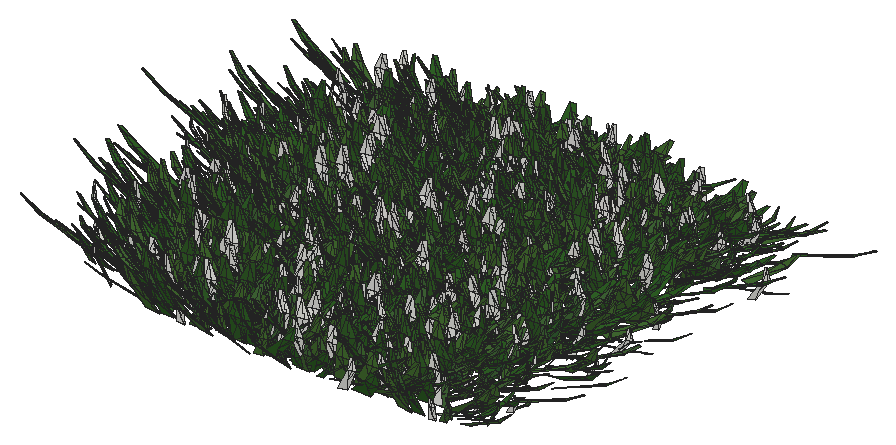
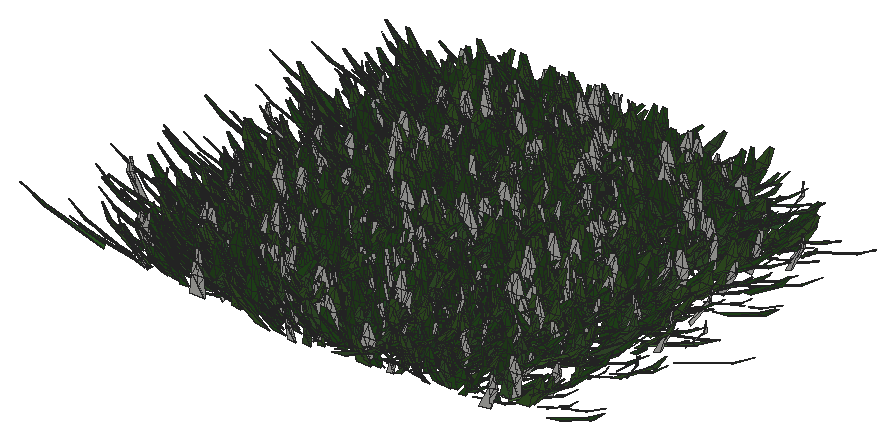
# SketchUp Ruby script. Lengths in inches.
U = 1.inch
M = Sketchup.active_model
def pt(a) = Geom::Point3d.new(a.map { |v| v * U })
def face(e, loops, mat)
  f = e.add_face(loops[0].map { |a| pt(a) })
  loops[1..].each { |l| e.add_face(l.map { |a| pt(a) }).erase! }
  f.material = f.back_material = mat if mat
  f
end
# faces: each face lists its corners as indices into pts; further lists are holes
def faces(e, pts, list, mat = nil) = list.each { |f| face(e, (f[0].is_a?(Array) ? f : [f]).map { |l| l.map { |i| pts[i] } }, mat) }
# xy, xz, yz: faces in a plane at the given z, y or x. An outline is a flat list of corners, or four numbers for a rectangle; further outlines are holes
def ring(l) = l.size == 4 ? [[l[0], l[1]], [l[2], l[1]], [l[2], l[3]], [l[0], l[3]]] : l.each_slice(2).to_a
def flat(e, list, mat, &to3) = list.each { |f| face(e, (f[0].is_a?(Array) ? f : [f]).map { |l| ring(l).map { |u, v| to3.(u, v) } }, mat) }
def xy(e, z, list, mat = nil) = flat(e, list, mat) { |x, y| [x, y, z] }
def xz(e, y, list, mat = nil) = flat(e, list, mat) { |x, z| [x, y, z] }
def yz(e, x, list, mat = nil) = flat(e, list, mat) { |y, z| [x, y, z] }
def lines(e, pts, list) = list.each { |a, b| e.add_line(pt(pts[a]), pt(pts[b])) }
# prism: a flat outline (further loops are holes) pulled along v
def prism(e, loops, v, mat = nil)
  f = face(e, loops, mat); d = Geom::Vector3d.new(v.map { |x| x * U })
  f.pushpull(f.normal.samedirection?(d) ? d.length : -d.length)
end
def box(e, o, s, mat = nil) = prism(e, [[o, [o[0] + s[0], o[1], o[2]], [o[0] + s[0], o[1] + s[1], o[2]], [o[0], o[1] + s[1], o[2]]]], [0, 0, s[2]], mat)
def at(x, y, z, deg = 0) = Geom::Transformation.translation(pt([x, y, z])) * Geom::Transformation.rotation(ORIGIN, Z_AXIS, deg.degrees)
def axes(o, x, y, z) = Geom::Transformation.new([*x, 0, *y, 0, *z, 0, *pt(o).to_a, 1])
def part(name) = M.definitions.add(name)
# library, detail: a bought-in or finely detailed component or shape, given as its bounding box
def library(name, o, s) = part(name).tap { |d| box(d.entities, o, s) }
def detail(e, o, s) = box(e.add_group.entities, o, s)
def put(e, d, t, mat = nil) = e.add_instance(d, t).tap { |i| i.material = mat if mat }
def group(e, t, mat = nil) = e.add_group.tap { |g| g.transformation = t; g.material = mat if mat }.entities
root = M.entities
M.materials.add("Material10").color = [48, 100, 38]
M.materials.add("Material3").color = [68, 110, 58]
M.materials.add("Material4").color = [48, 90, 38]
M.materials.add("Material5").color = [68, 110, 48]
M.materials.add("Material6").color = [48, 90, 48]
M.materials.add("Material7").color = [58, 110, 58]
M.materials.add("Material8").color = [58, 90, 38]
M.materials.add("Material9").color = [68, 100, 58]
c1 = part("grass00")
p = [[-0.6875,0.15,0],[-0.56,0.08,5.52],[-0.04,0.03,2.76],[0.48,-0.02,0],[0.35,-0.02,5.52],[-0.1,-0.14,5.52],
  [-0.12,0.65,8.37],[-0.42,0.65,8.37]]
faces(c1.entities,p,[[0,1,2,3],[3,2,4],[1,5,2],[5,4,2],[1,6,5],[4,5,6],[7,6,1]])
c2 = part("Group16\#1")
put(c2.entities,c1,axes([1.44,-0.61,-0.01],[0.05352,0.12609,0],[-0.10704,0.04543,0.07239],[0.06664,-0.02828,0.11628]),"Material6")
put(c2.entities,c1,axes([0.76,-0.15,-0.01],[0.04676,0.24062,0],[-0.23162,0.04501,0.06642],[0.0652,-0.01267,0.23595]),"Material3")
put(c2.entities,c1,axes([0.79,0.01,-0.01],[-0.00606,0.34651,0],[-0.34381,-0.00602,0.0432],[0.04319,0.00076,0.34386]))
put(c2.entities,c1,axes([1,0.23,-0.01],[-0.07192,0.31144,0],[-0.28722,-0.06632,0.1236],[0.12043,0.02781,0.29478]),"Material5")
put(c2.entities,c1,axes([1.66,0.77,-0.01],[-0.13828,0.29651,0],[-0.21551,-0.1005,0.22471],[0.20365,0.09498,0.23779]),"Material10")
put(c2.entities,c1,axes([0.6875,0.52,-0.01],[-0.18126,0.24051,0],[-0.22746,-0.17142,0.09788],[0.07817,0.05891,0.28481]),"Material5")
put(c2.entities,c1,axes([0.68,0.78,-0.01],[-0.215,0.18688,0],[-0.12385,-0.14248,0.21334],[0.13995,0.16101,0.18878]),"Material3")
put(c2.entities,c1,axes([0.56,1,-0.01],[-0.13756,0.07624,0],[-0.06159,-0.11112,0.0927],[0.04494,0.08108,0.12705]),"Material5")
put(c2.entities,c1,axes([0.2,0.64,-0.01],[-0.23729,0.07254,0],[-0.05711,-0.18681,0.153],[0.04473,0.14632,0.19535]),"Material10")
put(c2.entities,c1,axes([0.0625,0.72,-0.01],[-0.28874,0.02525,0],[-0.02179,-0.24916,0.14647],[0.01276,0.14591,0.25012]),"Material3")
put(c2.entities,c1,axes([-0.08,0.62,-0.01],[-0.34089,-0.04187,0],[0.03255,-0.26504,0.216],[-0.02633,0.21439,0.26703]),"Material10")
put(c2.entities,c1,axes([-0.34,0.98,-0.01],[-0.14314,-0.0493,0],[0.04397,-0.12769,0.06843],[-0.02228,0.0647,0.13505]),"Material10")
put(c2.entities,c1,axes([-0.87,1.45,-0.01],[-0.23488,-0.14114,0],[0.13761,-0.22901,0.06087],[-0.03135,0.05217,0.26717]))
put(c2.entities,c1,axes([-0.72,0.77,-0.01],[-0.14208,-0.13251,0],[0.07209,-0.0773,0.16301],[-0.11118,0.11922,0.1057]),"Material10")
put(c2.entities,c1,axes([-0.62,0.43,-0.01],[-0.14845,-0.21203,0],[0.18654,-0.13061,0.12304],[-0.10079,0.07057,0.22772]),"Material3")
put(c2.entities,c1,axes([-0.68,0.29,-0.01],[-0.13639,-0.32136,0],[0.31723,-0.13464,0.05579],[-0.05136,0.0218,0.34462]),"Material4")
put(c2.entities,c1,axes([-0.64,0.125,-0.01],[-0.0458,-0.23569,0],[0.22124,-0.043,0.08276],[-0.08124,0.01579,0.22538]),"Material7")
put(c2.entities,c1,axes([-1.6,-0.03,-0.01],[0.00576,-0.32897,0],[0.27526,0.00482,0.18018],[-0.18015,-0.00315,0.2753]),"Material5")
put(c2.entities,c1,axes([-1.36,-0.31,-0.01],[0.05718,-0.24765,0],[0.18172,0.04196,0.17267],[-0.16825,-0.03885,0.1865]),"Material10")
put(c2.entities,c1,axes([-1.54,-0.72,-0.01],[0.06537,-0.14017,0],[0.13555,0.06321,0.03939],[-0.0357,-0.01665,0.14956]))
put(c2.entities,c1,axes([-1.19,-0.9,-0.01],[0.09597,-0.12735,0],[0.11214,0.08451,0.07557],[-0.06035,-0.04548,0.14042]),"Material9")
put(c2.entities,c1,axes([-0.47,-0.54,-0.01],[0.11588,-0.10072,0],[0.0618,0.0711,0.12124],[-0.07953,-0.0915,0.0942]))
put(c2.entities,c1,axes([-0.47,-0.84,-0.01],[0.11927,-0.0661,0],[0.06603,0.11913,0.00646],[-0.00313,-0.00565,0.13621]),"Material5")
put(c2.entities,c1,axes([-0.38,-1.24,-0.01],[0.28037,-0.08571,0],[0.0618,0.20215,0.20315],[-0.05939,-0.19428,0.21139]),"Material9")
put(c2.entities,c1,axes([-0.06,-0.66,-0.01],[0.22719,-0.01987,0],[0.01247,0.14255,0.17758],[-0.01547,-0.17691,0.1431]),"Material8")
put(c2.entities,c1,axes([0.11,-0.89,-0.01],[0.14882,0.01828,0],[-0.01058,0.08611,0.12229],[0.01491,-0.12138,0.08676]),"Material6")
put(c2.entities,c1,axes([0.25,-0.72,-0.01],[0.20481,0.07053,0],[-0.06206,0.18022,0.10291],[0.03351,-0.0973,0.1906]),"Material6")
put(c2.entities,c1,axes([0.85,-1.42,-0.01],[0.16481,0.09904,0],[-0.09472,0.15762,0.05616],[0.02893,-0.04814,0.18389]),"Material5")
put(c2.entities,c1,axes([1.01,-1.09,-0.01],[0.21858,0.20385,0],[-0.17495,0.1876,0.15339],[0.10462,-0.11218,0.25652]),"Material10")
put(c2.entities,c1,axes([1.01,-0.71,-0.01],[0.08733,0.12473,0],[-0.06445,0.04512,0.13037],[0.1068,-0.07477,0.07867]),"Material6")
c3 = part("Group15\#1")
put(c3.entities,c2,at(0,0,0))
c4 = part("3darcstudiotree_grass00\#1")
put(c4.entities,c3,at(0,0,0))
put(root,c4,axes([159.55,67.09,7.6],[-4.17134,0.59694,0],[-1.91655,-0.83704,-0.03218],[-0.1099,-0.048,1.65786]))
put(root,c4,axes([160.14,46.88,7.6],[1.82974,-1.11236,0],[4.14269,0.4259,-0.00107],[0.00497,0.00051,1.41133]))
put(root,c4,axes([159.38,79.67,7.6],[-2.1717,0.94775,0],[-3.61053,-0.51708,-0.00674],[-0.03293,-0.00472,1.46389]))
put(root,c4,axes([159.7,53.77,7.6],[-1.78952,0.96069,0],[-3.60864,-0.42012,-0.01596],[-0.10849,-0.01263,1.86544]))
put(root,c4,axes([159.95,57.98,7.6],[-2.06309,0.87153,0],[-4.13288,-0.61146,-0.04665],[-0.19777,-0.02926,1.47851]))
put(root,c4,axes([161.13,74.04,7.6],[-3.51429,-0.45659,0],[1.66461,-0.80077,-0.02241],[0.07721,-0.03714,1.68548]))
put(root,c4,axes([160.16,66.55,7.6],[2.73197,0.7121,0],[-2.97454,0.71324,-0.02632],[-0.14399,0.03453,1.95302]))
put(root,c4,axes([160.55,71.85,7.6],[4.48019,-0.41485,0],[1.31658,0.88866,-0.03178],[0.08406,0.05674,1.80429]))
put(root,c4,axes([160.35,49.35,7.6],[2.54094,0.64898,0],[-3.14239,0.76896,-0.01876],[-0.08636,0.02113,1.77063]))
put(root,c4,axes([161.15,62.51,7.6],[0.1997,1.06432,0],[-4.51312,0.05293,-0.04808],[-0.29009,0.0034,1.70557]))
put(root,c4,axes([160.55,64.97,7.6],[1.85724,1.07697,0],[-4.66485,0.50278,-0.01792],[-0.06948,0.00749,1.34035]))
put(root,c4,axes([163.5,73.8125,7.6],[-1.0135,-1.00462,0],[4.08606,-0.25764,-0.02503],[0.13624,-0.00859,1.47852]))
put(root,c4,axes([162.99,53.55,7.6],[-4.005,0.7272,0],[-2.3018,-0.79231,-0.02785],[-0.12344,-0.04249,1.84622]))
put(root,c4,axes([162.97,61.53,7.6],[2.95335,-0.82152,0],[2.70823,0.6085,-0.01288],[0.06524,0.01466,1.54961]))
put(root,c4,axes([163.93,56.8125,7.6],[-4.20956,-0.26717,0],[1.18231,-1.16431,-0.00944],[0.01496,-0.01473,1.93444]))
put(root,c4,axes([163.76,52.31,7.6],[-1.13661,-1.06386,0],[4.15271,-0.27729,-0.04991],[0.23787,-0.01588,1.32514]))
put(root,c4,axes([163.9,51.05,7.6],[2.16693,-1.10955,0],[3.94511,0.48154,-0.03421],[0.21213,0.02589,1.89316]))
put(root,c4,axes([163.04,63.26,7.6],[1.18,1.03822,0],[-4.57121,0.32472,-0.01918],[-0.11705,0.00831,1.88463]))
put(root,c4,axes([164.6875,72.41,7.6],[-3.50507,0.61445,0],[-2.29769,-0.81919,-0.04222],[-0.17037,-0.06074,1.75818]))
put(root,c4,axes([165.76,69.23,7.6],[-3.58509,-0.60969,0],[2.592,-0.9526,-0.01911],[0.04957,-0.01822,1.32815]))
put(root,c4,axes([165.39,49.4,7.6],[-0.06451,-0.92143,0],[4.54272,-0.01988,-0.04239],[0.21245,-0.00093,1.42343]))
put(root,c4,axes([165.45,74.96,7.6],[-4.03446,-0.01635,0],[0.06659,-1.02672,-0.00434],[0.00038,-0.00582,1.37632]))
put(root,c4,axes([164.02,81.125,7.6],[3.92463,0.27646,0],[-1.34669,1.19487,-0.04858],[-0.06681,0.05928,1.57379]))
put(root,c4,axes([166.28,60.26,7.6],[-0.14207,-1.06089,0],[4.63971,-0.03883,-0.02714],[0.13515,-0.00113,1.44559]))
put(root,c4,axes([165.8,66.5,7.6],[-4.11295,0.48392,0],[-1.88318,-1.00036,-0.0027],[-0.00657,-0.00349,1.57765]))
put(root,c4,axes([165.86,79.88,7.6],[-3.01374,0.50325,0],[-2.28022,-0.85345,-0.04884],[-0.14675,-0.05493,1.38796]))
put(root,c4,axes([165.86,45.25,7.6],[2.85144,-0.93309,0],[3.29337,0.62902,-0.00592],[0.03247,0.0062,1.78738]))
put(root,c4,axes([166.8,45.98,7.6],[-2.85912,-0.7944,0],[3.18267,-0.71592,-0.02928],[0.11058,-0.02487,1.35967]))
put(root,c4,axes([167.0625,77.8,7.6],[-4.01975,-0.67401,0],[2.06418,-0.76941,-0.03319],[0.1306,-0.04868,1.63594]))
put(root,c4,axes([165.64,70.24,7.6],[-0.9226,1.08456,0],[-4.51637,-0.24012,-0.02719],[-0.16539,-0.00879,1.79436]))
put(root,c4,axes([165.94,64.02,7.6],[-0.15668,0.99341,0],[-4.74141,-0.04674,-0.01193],[-0.07952,-0.00078,1.97773]))
put(root,c4,axes([166.9,67.77,7.6],[-0.75974,1.09038,0],[-3.60462,-0.15698,-0.03897],[-0.29833,-0.01299,1.77692]))
put(root,c4,axes([166.78,55.85,7.6],[-0.10594,0.90385,0],[-3.73304,-0.02735,-0.04664],[-0.28296,-0.00207,1.41669]))
put(root,c4,axes([166.32,43.64,7.6],[1.08855,0.96574,0],[-4.18203,0.29461,-0.02067],[-0.12416,0.00875,1.69495]))
put(root,c4,axes([166.72,59,7.6],[3.05692,0.87665,0],[-2.75486,0.6004,-0.0286],[-0.17096,0.03726,1.81122]))
put(root,c4,axes([166.99,48.17,7.6],[-0.61059,1.1553,0],[-4.99702,-0.16506,-0.03274],[-0.14868,-0.00491,1.44297]))
put(root,c4,axes([166.8125,76.65,7.6],[4.02977,0.69816,0],[-2.76519,0.99754,-0.01195],[-0.03084,0.01113,1.37528]))
put(root,c4,axes([169.07,69.11,7.6],[-4.6224,0.20326,0],[-0.67084,-0.9535,-0.03096],[-0.03075,-0.04371,1.38775]))
put(root,c4,axes([169.28,58.54,7.6],[-3.52473,0.27582,0],[-1.46531,-1.17033,-0.0251],[-0.03902,-0.03117,1.59541]))
put(root,c4,axes([169.85,79.63,7.6],[-3.34559,-0.54215,0],[2.26075,-0.87194,-0.04254],[0.15941,-0.06148,1.78955]))
put(root,c4,axes([169.31,67.16,7.6],[-3.01586,0.58588,0],[-3.13511,-1.00864,-0.03993],[-0.14863,-0.04782,1.9372]))
put(root,c4,axes([170.27,71.76,7.6],[-4.50764,0.05804,0],[-0.237,-1.15033,-0.00589],[-0.00143,-0.00694,1.35922]))
put(root,c4,axes([169.34,49,7.6],[0.84914,1.0367,0],[-4.55233,0.23304,-0.02758],[-0.15102,0.00773,1.62317]))
put(root,c4,axes([171.27,81.41,7.6],[0.34339,-1.17076,0],[3.77324,0.06917,-0.00239],[0.01439,0.00026,1.42634]))
put(root,c4,axes([169.63,59.57,7.6],[0.91899,1.10711,0],[-4.12174,0.21384,-0.00381],[-0.02297,0.00119,1.62105]))
put(root,c4,axes([171.51,75.35,7.6],[-4.49867,-0.03279,0],[0.10809,-0.92683,-0.0193],[0.00484,-0.04152,1.99558]))
put(root,c4,axes([171.56,55.1,7.6],[-5.14292,0.15234,0],[-0.50377,-1.06293,-0.03012],[-0.01728,-0.03646,1.30483]))
put(root,c4,axes([170.37,46.2,7.6],[-1.72517,0.88368,0],[-4.30295,-0.52503,-0.02753],[-0.1522,-0.01857,1.84121]))
put(root,c4,axes([170.79,48.26,7.6],[2.2537,-0.76087,0],[3.152,0.58351,-0.04843],[0.27401,0.05073,1.72564]))
put(root,c4,axes([171.55,77.66,7.6],[0.63611,-1.02473,0],[3.70027,0.14356,-0.00401],[0.03085,0.0012,1.82024]))
put(root,c4,axes([171.91,61.68,7.6],[1.35745,-0.83433,0],[3.74558,0.38088,-0.0011],[0.00732,0.00074,1.80895]))
put(root,c4,axes([171.97,53.8,7.6],[0.97823,-1.25703,0],[4.41558,0.21476,-0.02432],[0.13179,0.00641,1.55217]))
put(root,c4,axes([172.9375,52.29,7.6],[0.22032,-0.95228,0],[4.21041,0.06088,-0.03098],[0.18429,0.00266,1.57088]))
put(root,c4,axes([173.47,64.89,7.6],[-3.97708,-0.65638,0],[2.24406,-0.84981,-0.0411],[0.12771,-0.04836,1.43569]))
put(root,c4,axes([173.32,51.44,7.6],[-0.40729,-1.01292,0],[4.15369,-0.10439,-0.02999],[0.21852,-0.00549,1.91089]))
put(root,c4,axes([171.97,43.42,7.6],[4.502,0.00283,0],[-0.01155,1.14774,-0.01268],[-0.0002,0.02022,1.83013]))
put(root,c4,axes([173.02,62.72,7.6],[2.20159,-0.97329,0],[4.02139,0.56853,-0.04614],[0.20661,0.02921,1.48544]))
put(root,c4,axes([173.05,44.41,7.6],[3.52289,-0.91079,0],[3.16711,0.76564,-0.03201],[0.1577,0.03812,1.88682]))
put(root,c4,axes([172.56,73.99,7.6],[4.48262,0.00833,0],[-0.03164,1.06491,-0.04293],[-0.00162,0.05463,1.35522]))
put(root,c4,axes([173.08,65.51,7.6],[3.85076,-0.25069,0],[1.03247,0.9912,-0.03218],[0.04181,0.04014,1.32043]))
put(root,c4,axes([173.3125,70.56,7.6],[3.89613,-0.16105,0],[0.82507,1.24749,-0.01648],[0.01292,0.01954,1.51991]))
put(root,c4,axes([173.46,77.04,7.6],[-0.04726,1.09729,0],[-5.17965,-0.01394,-0.05791],[-0.28781,-0.00077,1.60897]))
put(root,c4,axes([173.29,56.47,7.6],[5.05688,0.26305,0],[-1.05641,1.26926,-0.01168],[-0.01025,0.01231,1.39591]))
put(root,c4,axes([175.7,44.27,7.6],[2.70054,-0.71079,0],[3.38542,0.8039,-0.03691],[0.17495,0.04154,1.90749]))
put(root,c4,axes([176.76,60.24,7.6],[-3.16844,-0.68398,0],[2.56496,-0.74262,-0.01919],[0.10195,-0.02952,1.99409]))
put(root,c4,axes([175,81.52,7.6],[5.10235,-0.04118,0],[0.1288,0.99748,-0.01793],[0.00416,0.0322,1.79317]))
put(root,c4,axes([177.03,49.89,7.6],[-3.29965,-0.97084,0],[3.65156,-0.77567,-0.06095],[0.27313,-0.05802,1.76096]))
put(root,c4,axes([176.86,75.44,7.6],[0.00475,-1.00888,0],[4.13099,0.00122,-0.01884],[0.10616,0.00003,1.45492]))
put(root,c4,axes([176.86,52.78,7.6],[1.28562,-1.04456,0],[4.88305,0.37562,-0.02541],[0.11276,0.00867,1.48254]))
put(root,c4,axes([176.84,76.73,7.6],[-4.01095,0.48354,0],[-1.72258,-0.89306,-0.02015],[-0.06662,-0.03454,1.88684]))
put(root,c4,axes([177.625,56.91,7.6],[-4.2659,-0.35222,0],[1.33923,-1.01376,-0.04962],[0.10523,-0.07966,1.8049]))
put(root,c4,axes([176.94,51.29,7.6],[-3.11352,0.45479,0],[-2.39689,-1.02558,-0.05376],[-0.12618,-0.05399,1.38154]))
put(root,c4,axes([176.4,58.78,7.6],[-1.0061,1.18777,0],[-4.7987,-0.25405,-0.05285],[-0.29037,-0.01537,1.72177]))
put(root,c4,axes([178.01,82.32,7.6],[-1.74766,-0.79325,0],[4.51404,-0.62157,-0.06742],[0.28979,-0.0399,1.58058]))
put(root,c4,axes([177.23,64.4375,7.6],[-3.06069,0.9303,0],[-3.81711,-0.78489,-0.01702],[-0.08141,-0.01674,1.91367]))
put(root,c4,axes([177,79.29,7.6],[4.53702,-0.3939,0],[1.61159,1.16016,-0.03586],[0.06911,0.04975,1.80381]))
put(root,c4,axes([177.2,46.51,7.6],[4.54274,-0.04809,0],[0.18784,1.10891,-0.02002],[0.00517,0.03055,1.69539]))
put(root,c4,axes([178.63,72.29,7.6],[-4.54396,0.24782,0],[-0.94268,-1.08027,-0.03649],[-0.05075,-0.05815,1.80375]))
put(root,c4,axes([177.18,68.8,7.6],[4.69542,0.51602,0],[-1.76105,1.00152,-0.02572],[-0.05567,0.03166,1.47108]))
put(root,c4,axes([179.125,42.98,7.6],[-3.49013,-0.33538,0],[1.59635,-1.03827,-0.04802],[0.0959,-0.06237,1.54794]))
put(root,c4,axes([179.23,55.01,7.6],[-4.19082,-0.16381,0],[0.77881,-1.24532,-0.04342],[0.03554,-0.05683,1.66984]))
put(root,c4,axes([178.06,62.81,7.6],[-2.14588,1.16725,0],[-4.21362,-0.48414,-0.02861],[-0.16909,-0.01943,1.88512]))
put(root,c4,axes([179.06,66.49,7.6],[-0.93459,-0.91429,0],[3.85666,-0.24639,-0.03508],[0.2611,-0.01668,1.91126]))
put(root,c4,axes([179.29,53.46,7.6],[-3.7798,-0.05998,0],[0.31505,-1.24085,-0.04372],[0.01169,-0.04605,1.31241]))
put(root,c4,axes([178.83,67.92,7.6],[-2.07802,0.79254,0],[-3.06125,-0.50166,-0.04],[-0.21333,-0.03496,1.45882]))
put(root,c4,axes([179.44,73.74,7.6],[-4.99575,0.35243,0],[-1.3345,-1.18231,-0.00145],[-0.00235,-0.00208,1.8291]))
put(root,c4,axes([178.22,78.52,7.6],[-0.1036,1.25235,0],[-5.07637,-0.02625,-0.04199],[-0.22282,-0.00115,1.68448]))
put(root,c4,axes([178.5,70.37,7.6],[4.03192,-0.06171,0],[0.31158,1.27245,-0.0507],[0.01617,0.06605,1.66388]))
put(root,c4,axes([178.63,61.47,7.6],[1.41099,1.21427,0],[-3.49838,0.25407,-0.00931],[-0.0535,0.00389,1.3628]))
put(root,c4,axes([179.47,48.36,7.6],[3.54443,-0.39661,0],[1.7308,0.96674,-0.04939],[0.13763,0.07687,1.80606]))
put(root,c4,axes([181.27,67.74,7.6],[-3.31485,0.87666,0],[-3.1697,-0.74909,-0.01805],[-0.08242,-0.01948,1.71251]))
put(root,c4,axes([181.77,63.21,7.6],[-3.48936,0.44199,0],[-1.76039,-0.8686,-0.00642],[-0.01577,-0.00778,1.3229]))
put(root,c4,axes([182.45,46.23,7.6],[-3.90886,-0.30229,0],[1.49188,-1.20572,-0.06046],[0.08426,-0.0681,1.48798]))
put(root,c4,axes([181.6,70.03,7.6],[-2.47789,0.67823,0],[-3.79555,-0.86668,-0.00484],[-0.01733,-0.00396,1.55938]))
put(root,c4,axes([181.95,44.7,7.6],[-3.37517,0.74484,0],[-3.41277,-0.96654,-0.01862],[-0.07294,-0.02066,1.90809]))
put(root,c4,axes([183.24,65.93,7.6],[-1.16922,-0.89242,0],[4.84591,-0.39681,-0.01545],[0.0714,-0.00585,1.54954]))
put(root,c4,axes([183.3,43.74,7.6],[-0.55416,-0.96725,0],[5.02165,-0.17981,-0.00214],[0.01069,-0.00038,1.59988]))
put(root,c4,axes([181.92,57.19,7.6],[-2.38604,0.77212,0],[-3.59178,-0.69372,-0.01374],[-0.06498,-0.01255,1.69563]))
put(root,c4,axes([181.55,49.59,7.6],[-1.2357,1.15486,0],[-4.4486,-0.2975,-0.00132],[-0.00824,-0.00055,1.858]))
put(root,c4,axes([181.12,61.59,7.6],[3.55659,0.85158,0],[-3.47186,0.90625,-0.01961],[-0.07165,0.0187,1.65716]))
put(root,c4,axes([183.15,47.77,7.6],[-4.00701,0.12184,0],[-0.61913,-1.27256,-0.00408],[-0.00269,-0.00553,1.74968]))
put(root,c4,axes([181.6,77.15,7.6],[0.70953,1.23995,0],[-4.73718,0.16942,-0.02596],[-0.11397,0.00408,1.32635]))
put(root,c4,axes([181.83,64.03,7.6],[-1.18063,1.19799,0],[-4.72808,-0.29122,-0.00818],[-0.04761,-0.00293,1.82396]))
put(root,c4,axes([182.17,78.31,7.6],[2.66838,1.01095,0],[-3.09046,0.50982,-0.04277],[-0.24475,0.04038,1.58679]))
put(root,c4,axes([182.88,72.5,7.6],[4.51633,0.0703,0],[-0.2535,1.0179,-0.04181],[-0.01988,0.07984,1.95138]))
put(root,c4,axes([184.22,80.68,7.6],[-3.87975,0.70385,0],[-2.42692,-0.83611,-0.01293],[-0.05657,-0.01949,1.92389]))
put(root,c4,axes([182.85,59.51,7.6],[3.24301,0.83296,0],[-3.40593,0.82878,-0.004],[-0.01826,0.00444,1.89371]))
put(root,c4,axes([184.82,52.76,7.6],[-4.54194,0.17936,0],[-0.65445,-1.03581,-0.01239],[-0.01049,-0.01661,1.42361]))
put(root,c4,axes([183.45,50.95,7.6],[4.6124,0.10308,0],[-0.35679,0.99786,-0.01038],[-0.00716,0.02002,1.94021]))
put(root,c4,axes([183.46,69.04,7.6],[4.49423,0.49278,0],[-1.72551,0.98355,-0.04488],[-0.1327,0.07564,1.97665]))
put(root,c4,axes([183.6,54.17,7.6],[1.21551,1.05496,0],[-3.93123,0.28309,-0.02733],[-0.16885,0.01216,1.64375]))
put(root,c4,axes([184.73,79.375,7.6],[2.41626,-0.681,0],[3.66998,0.81384,-0.037],[0.13802,0.03061,1.52862]))
put(root,c4,axes([184.61,75.1875,7.6],[2.63621,0.70043,0],[-2.68447,0.63147,-0.04643],[-0.25687,0.06042,1.7498]))
put(root,c4,axes([184.61,73.89,7.6],[2.03725,0.93622,0],[-3.24747,0.44167,-0.01685],[-0.12399,0.01686,1.93576]))
put(root,c4,axes([184.89,59.03,7.6],[4.58865,0.50519,0],[-1.59978,0.90817,-0.04159],[-0.09607,0.05454,1.42181]))
put(root,c4,axes([187.125,50.44,7.6],[-2.01574,-1.10957,0],[4.29176,-0.4873,-0.02239],[0.13134,-0.01491,1.89813]))
put(root,c4,axes([185.51,55.06,7.6],[1.09378,1.21386,0],[-4.24535,0.23909,-0.04632],[-0.26606,0.01498,1.6013]))
put(root,c4,axes([187.63,70.76,7.6],[-4.678,-0.23812,0],[0.97178,-1.1932,-0.03896],[0.04515,-0.05543,1.76791]))
put(root,c4,axes([187.29,69.47,7.6],[3.3432,-0.58816,0],[2.82496,1.00359,-0.04926],[0.17837,0.06337,1.93034]))
put(root,c4,axes([187.61,73.31,7.6],[-3.21056,0.58828,0],[-2.88924,-0.98552,-0.02359],[-0.07623,-0.026,1.66971]))
put(root,c4,axes([188.77,80.25,7.6],[-4.42597,-0.65302,0],[1.92536,-0.81559,-0.01139],[0.03728,-0.01579,1.52439]))
put(root,c4,axes([188.9,46.15,7.6],[-0.4988,-1.1669,0],[3.78624,-0.10115,-0.01446],[0.09735,-0.0026,1.61179]))
put(root,c4,axes([188.29,45.22,7.6],[-3.42941,0.55901,0],[-2.40319,-0.92143,-0.02083],[-0.06645,-0.02548,1.60618]))
put(root,c4,axes([189.28,77.81,7.6],[-4.16493,-0.30995,0],[1.21489,-1.02032,-0.0137],[0.02048,-0.0172,1.39479]))
put(root,c4,axes([189.67,60.06,7.6],[-3.70141,-0.8816,0],[3.55908,-0.93393,-0.03405],[0.10659,-0.02797,1.46358]))
put(root,c4,axes([187.51,54.4,7.6],[1.53914,1.0513,0],[-4.39566,0.40221,-0.03042],[-0.15696,0.01436,1.60735]))
put(root,c4,axes([187.98,64.38,7.6],[4.38638,0.43915,0],[-1.65781,1.03492,-0.05201],[-0.12203,0.07618,1.75905]))
put(root,c4,axes([189.03,76.69,7.6],[3.5333,-0.35922,0],[1.45173,0.89244,-0.02601],[0.05982,0.03677,1.4702]))
put(root,c4,axes([188.76,72.08,7.6],[4.6185,-0.19049,0],[0.64707,0.98053,-0.03976],[0.0459,0.06956,1.7619]))
put(root,c4,axes([189.27,49.41,7.6],[-0.10897,1.07036,0],[-4.26555,-0.02714,-0.03168],[-0.19713,-0.00125,1.66016]))
put(root,c4,axes([189.86,61.67,7.6],[3.42773,-0.49366,0],[2.33187,1.01196,-0.00508],[0.01362,0.00591,1.56982]))
put(root,c4,axes([189.39,58.67,7.6],[1.88253,1.20428,0],[-4.05103,0.39579,-0.05423],[-0.25457,0.02487,1.37014]))
put(root,c4,axes([190.95,55.52,7.6],[1.67023,-1.19421,0],[4.03376,0.3526,-0.01723],[0.08743,0.00764,1.43549]))
put(root,c4,axes([190.46,48.18,7.6],[-2.65738,1.09384,0],[-4.1127,-0.62446,-0.06137],[-0.25477,-0.03868,1.46064]))
put(root,c4,axes([190.11,52.09,7.6],[3.93411,-0.32217,0],[1.27665,0.97436,-0.03684],[0.07239,0.05525,1.61813]))
put(root,c4,axes([190.35,81.08,7.6],[4.66298,-0.3319,0],[1.18544,1.04091,-0.0361],[0.05479,0.04811,1.4995]))
put(root,c4,axes([191.37,56.61,7.6],[-3.31735,0.93033,0],[-2.98242,-0.66466,-0.02096],[-0.10528,-0.02346,1.6805]))
put(root,c4,axes([191.22,67.12,7.6],[-1.67728,0.97063,0],[-4.3061,-0.46507,-0.05011],[-0.26514,-0.02864,1.6899]))
put(root,c4,axes([191.61,65.56,7.6],[-2.6954,0.74968,0],[-3.20953,-0.72123,-0.05045],[-0.20663,-0.04643,1.48531]))
put(root,c4,axes([191.08,75.04,7.6],[0.74763,1.2665,0],[-3.58863,0.1324,-0.00575],[-0.0331,0.00122,1.31904]))
put(root,c4,axes([191.29,43.63,7.6],[0.50371,0.92792,0],[-3.91618,0.13287,-0.02967],[-0.18729,0.00635,1.57371]))
put(root,c4,axes([193.4,74.17,7.6],[-3.39734,-0.81214,0],[3.21264,-0.83994,-0.00934],[0.03489,-0.00912,1.57129]))
